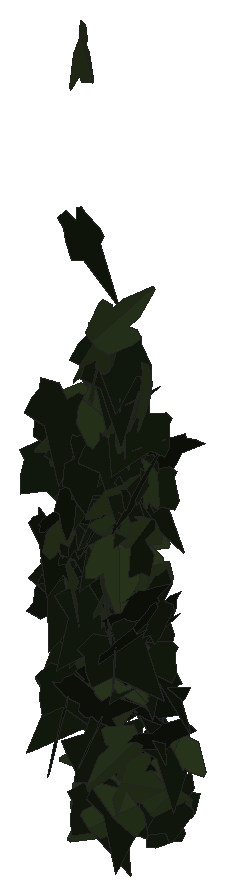
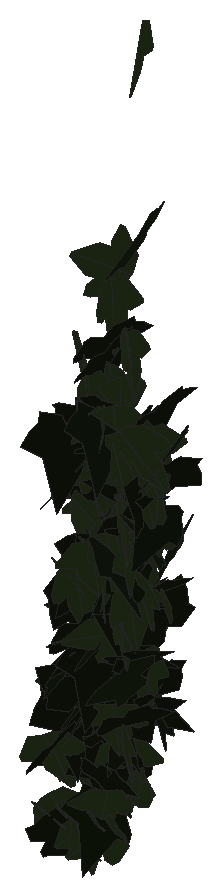
# SketchUp Ruby script. Lengths in inches.
U = 1.inch
M = Sketchup.active_model
def pt(a) = Geom::Point3d.new(a.map { |v| v * U })
def face(e, loops, mat)
  f = e.add_face(loops[0].map { |a| pt(a) })
  loops[1..].each { |l| e.add_face(l.map { |a| pt(a) }).erase! }
  f.material = f.back_material = mat if mat
  f
end
# faces: each face lists its corners as indices into pts; further lists are holes
def faces(e, pts, list, mat = nil) = list.each { |f| face(e, (f[0].is_a?(Array) ? f : [f]).map { |l| l.map { |i| pts[i] } }, mat) }
# xy, xz, yz: faces in a plane at the given z, y or x. An outline is a flat list of corners, or four numbers for a rectangle; further outlines are holes
def ring(l) = l.size == 4 ? [[l[0], l[1]], [l[2], l[1]], [l[2], l[3]], [l[0], l[3]]] : l.each_slice(2).to_a
def flat(e, list, mat, &to3) = list.each { |f| face(e, (f[0].is_a?(Array) ? f : [f]).map { |l| ring(l).map { |u, v| to3.(u, v) } }, mat) }
def xy(e, z, list, mat = nil) = flat(e, list, mat) { |x, y| [x, y, z] }
def xz(e, y, list, mat = nil) = flat(e, list, mat) { |x, z| [x, y, z] }
def yz(e, x, list, mat = nil) = flat(e, list, mat) { |y, z| [x, y, z] }
def lines(e, pts, list) = list.each { |a, b| e.add_line(pt(pts[a]), pt(pts[b])) }
# prism: a flat outline (further loops are holes) pulled along v
def prism(e, loops, v, mat = nil)
  f = face(e, loops, mat); d = Geom::Vector3d.new(v.map { |x| x * U })
  f.pushpull(f.normal.samedirection?(d) ? d.length : -d.length)
end
def box(e, o, s, mat = nil) = prism(e, [[o, [o[0] + s[0], o[1], o[2]], [o[0] + s[0], o[1] + s[1], o[2]], [o[0], o[1] + s[1], o[2]]]], [0, 0, s[2]], mat)
def at(x, y, z, deg = 0) = Geom::Transformation.translation(pt([x, y, z])) * Geom::Transformation.rotation(ORIGIN, Z_AXIS, deg.degrees)
def axes(o, x, y, z) = Geom::Transformation.new([*x, 0, *y, 0, *z, 0, *pt(o).to_a, 1])
def part(name) = M.definitions.add(name)
# library, detail: a bought-in or finely detailed component or shape, given as its bounding box
def library(name, o, s) = part(name).tap { |d| box(d.entities, o, s) }
def detail(e, o, s) = box(e.add_group.entities, o, s)
def put(e, d, t, mat = nil) = e.add_instance(d, t).tap { |i| i.material = mat if mat }
def group(e, t, mat = nil) = e.add_group.tap { |g| g.transformation = t; g.material = mat if mat }.entities
root = M.entities
M.materials.add("efeu1").color = [18, 25, 13]
M.materials.add("efeu2").color = [43, 57, 29]
c1 = part("ivyleaf_10")
p = [[0,0.5,-0.03],[-0.0625,2.02,-0.43],[-0.19,2.01,-0.46],[-0.54,1.05,-0.29],[-0.52,0.625,-0.18],[-0.83,0.76,-0.28],
  [-1.16,0.64,-0.33],[-1.15,0.33,-0.24],[-0.77,-0.39,0.02],[-0.3,-0.51,0.16],[0.04,-0.48,0.23],[-0.02,2.01,-0.4375],
  [-0.06,2.01,-0.43],[0.04,-0.49,0.23],[0.67,-0.49,0.14],[1.38,0.36,-0.2],[1.375,0.51,-0.24],[0.81,0.65,-0.19],
  [0.62,0.59,-0.15],[0.6,1.09,-0.28],[0.5,1.23,-0.31]]
faces(c1.entities,p,[[0,1,2,3,4,5,6,7,8,9,10],[11,12,0,13,14,15,16,17,18,19,20]],"efeu2")
c2 = part("ivyleaf_9")
p = [[1.54,2.16,1.25],[1.36,2.04,1.19],[-0.21,0.99,0.68],[-0.71,1.11,0.82],[-0.85,0.86,0.67],[-0.8,0.17,0.21],
  [-0.9,-0.01,0.1],[-0.67,-0.16,-0.02],[-0.08,-0.08,-0.05],[-0.03,-0.6,-0.4],[0.65,-0.88,-0.66],[0.83,-0.6,-0.49],
  [1.29,-0.42,-0.43],[1.8125,-0.07,-0.26],[1.21,0.44,0.15]]
faces(c2.entities,p,[[0,1,2,3,4,5,6,7,8,9,10,11,12,13,14]],"efeu1")
put(root,c1,axes([544.36,133.63,215.28],[0.76593,-0.47573,-0.00913],[0.0013,0.0194,-0.90149],[0.47582,0.76574,0.01717]))
put(root,c2,axes([544.35,134.4,210.57],[-0.44146,-0.74203,-0.00391],[0.04769,-0.02384,-0.86178],[0.7405,-0.44083,0.05318]))
put(root,c2,axes([543.96,132.84,219.55],[0.33357,-0.84112,0.18283],[0.07333,-0.16759,-0.90483],[0.85763,0.34148,0.00626]))
put(root,c1,axes([544.5625,133.91,214.71],[-0.18396,-0.86827,0.02169],[0.00495,-0.02321,-0.8875],[0.86853,-0.18377,0.00965]))
put(root,c2,axes([543.97,134.21,212.19],[0.76378,-0.42176,-0.05989],[0.10196,0.30037,-0.81499],[0.41361,0.70479,0.3115]))
put(root,c2,axes([544.15,132.43,215.58],[0.12089,-0.66184,0.61024],[0.07547,-0.6061,-0.6723],[0.89706,0.14019,-0.02568]))
put(root,c1,axes([544.85,133.55,220.17],[0.81777,0.15887,-0.54508],[-0.54725,-0.03404,-0.83094],[-0.15124,0.98219,0.05937]))
put(root,c2,axes([544.77,133.875,212.46],[-0.69047,-0.50333,0.18217],[-0.01066,-0.28433,-0.82602],[0.53518,-0.65505,0.21857]))
put(root,c2,axes([544.31,132.46,213.21],[-0.08317,-0.27642,0.86094],[0.76205,0.44397,0.21616],[-0.48674,0.74232,0.19131]))
put(root,c2,axes([544.72,132,217.1],[0.19383,0.78185,0.38972],[0.11374,0.37321,-0.8053],[-0.86616,0.22397,-0.01854]))
put(root,c1,axes([544.78,132.54,219.66],[-0.17417,-0.89754,0.09825],[-0.02854,-0.09454,-0.91423],[0.90245,-0.17621,-0.00995]))
put(root,c1,axes([544.98,132.62,211.78],[-0.85614,0.15785,0.30309],[-0.30004,0.04409,-0.87051],[-0.16356,-0.90713,0.01043]))
put(root,c2,axes([544.85,132.92,217.6],[0.05782,-0.11447,0.88511],[0.12882,0.87875,0.10523],[-0.88314,0.12069,0.0733]))
put(root,c2,axes([544.96,132.96,210.1],[-0.67636,-0.5024,0.20746],[-0.15286,-0.142,-0.84225],[0.52161,-0.69307,0.02218]))
put(root,c2,axes([544.39,132.33,218.87],[-0.09644,-0.71579,-0.59865],[0.14264,0.58346,-0.7206],[0.92217,-0.1651,0.04886]))
put(root,c1,axes([545.19,132.8,218.66],[-0.80348,-0.04527,0.45626],[-0.45087,-0.08926,-0.80284],[0.08331,-0.91966,0.05546]))
put(root,c2,axes([544.6875,132.9,214.22],[-0.29914,-0.82493,0.19051],[-0.01884,-0.19552,-0.87618],[0.84643,-0.29589,0.04783]))
put(root,c1,axes([544.74,132.17,216.39],[-0.06668,-0.76893,-0.42899],[0.26526,0.39269,-0.7451],[0.8396,-0.18513,0.20133]))
put(root,c2,axes([544.6875,132.37,210.19],[-0.42072,0.13063,-0.75248],[0.69411,-0.29297,-0.43895],[-0.31859,-0.8108,0.03738]))
put(root,c1,axes([544.93,133.96,209.78],[0.67624,-0.5645,-0.16398],[-0.10467,0.13032,-0.88029],[0.57844,0.68352,0.03241]))
put(root,c1,axes([544.78,134.39,210.59],[0.72269,0.46259,-0.0301],[-0.0271,-0.01349,-0.85806],[-0.46278,0.72319,0.00324]))
put(root,c1,axes([545.02,133.05,219.49],[-0.07678,-0.81983,0.38889],[-0.01917,-0.38872,-0.82327],[0.90718,-0.0776,0.01552]))
put(root,c2,axes([544.48,133.22,215.6875],[0.42107,-0.79258,-0.01396],[-0.01076,0.01009,-0.89748],[0.79263,0.42118,-0.00476]))
put(root,c1,axes([545,133.44,215.64],[-0.05752,-0.87897,-0.07927],[0.02266,0.07794,-0.88067],[0.88224,-0.05931,0.01745]))
put(root,c2,axes([544.74,132.31,211.1875],[0.10884,-0.57616,-0.64225],[-0.1346,0.62808,-0.58625],[0.85225,0.17278,-0.01057]))
put(root,c2,axes([544.75,132.31,220.81],[-0.04428,-0.92209,0.0919],[-0.01273,-0.09139,-0.92311],[0.92657,-0.04532,-0.00829]))
put(root,c1,axes([545.08,133.77,213.84],[0.26784,-0.85015,-0.09039],[-0.00354,0.09362,-0.89101],[0.85494,0.26673,0.02463]))
put(root,c1,axes([545.17,133.41,217.6],[0.24785,-0.82408,-0.29428],[-0.06142,0.28872,-0.86024],[0.87289,0.25431,0.02303]))
put(root,c2,axes([545.22,134.38,206.92],[0.27446,0.78455,0.18613],[-0.04767,0.21206,-0.82356],[-0.80492,0.25496,0.11224]))
put(root,c2,axes([545.52,133.95,216.19],[-0.56786,0.67413,-0.07436],[0.03608,-0.06682,-0.88129],[-0.67726,-0.56879,0.01539]))
put(root,c2,axes([544.86,132.83,212.32],[0.00984,-0.18546,0.87666],[0.64093,0.61414,0.12273],[-0.6262,0.62567,0.13939]))
put(root,c1,axes([544.58,132.39,214.32],[0.57667,-0.23355,0.67278],[0.65854,-0.15469,-0.61816],[0.27112,0.8725,0.07049]))
put(root,c2,axes([545.32,132.11,215.97],[-0.64082,0.64069,-0.17112],[-0.15267,0.08903,0.90508],[0.64533,0.65727,0.0442]))
put(root,c2,axes([544.84,133.26,215.51],[0.87645,-0.01594,-0.19155],[-0.18917,0.08691,-0.8728],[0.03406,0.89292,0.08154]))
put(root,c2,axes([545.02,133.65,217.5],[-0.25745,-0.84777,0.09368],[-0.01198,-0.09425,-0.88586],[0.85285,-0.25724,0.01584]))
put(root,c2,axes([545.25,134.58,208.4],[-0.7727,-0.20546,-0.31245],[0.30923,0.05222,-0.7991],[0.21027,-0.83184,0.02701]))
put(root,c1,axes([544.95,134.63,207.49],[0.53789,0.64418,0.14873],[0.10208,0.10851,-0.83917],[-0.65319,0.54742,-0.00867]))
put(root,c1,axes([544.96,133.61,215.96],[-0.64233,0.37563,-0.49597],[0.39211,-0.30905,-0.74189],[-0.48304,-0.75037,0.05728]))
put(root,c1,axes([545.02,132.83,217.82],[0.8416,0.13114,0.2751],[0.22307,0.28542,-0.8185],[-0.20765,0.83816,0.23568]))
put(root,c2,axes([545.33,133.57,213.62],[-0.48779,-0.73922,0.07842],[-0.02927,-0.07463,-0.8855],[0.74279,-0.48838,0.01661]))
put(root,c2,axes([545.74,132.59,209.23],[-0.31755,0.22971,-0.89619],[-0.69468,0.56659,0.39137],[0.61103,0.76353,-0.0208]))
put(root,c1,axes([544.91,134.52,206.15],[0.4604,0.15133,0.70044],[0.55774,0.44707,-0.46319],[-0.44994,0.70902,0.14256]))
put(root,c1,axes([545.67,132.85,208.19],[-0.68468,-0.53058,0.13792],[-0.10141,-0.09429,-0.86611],[0.53875,-0.69204,0.01226]))
put(root,c1,axes([545.51,133.18,219.44],[0.18367,-0.89419,-0.13502],[0.05585,0.14873,-0.90901],[0.9026,0.17275,0.08372]))
put(root,c1,axes([545.12,133.69,213.18],[0.01221,-0.03147,0.96719],[0.33212,0.90866,0.02537],[-0.90893,0.33159,0.02227]))
put(root,c1,axes([545.63,133.72,216.64],[-0.16809,-0.88289,0.05335],[0.01245,-0.05667,-0.89846],[0.88441,-0.167,0.02279]))
put(root,c2,axes([545.45,132.96,219.14],[-0.38516,-0.83459,-0.0298],[0.01269,0.02697,-0.91918],[0.83502,-0.38537,0.00022]))
put(root,c2,axes([545.62,131.37,218.44],[0.3081,-0.25107,-0.81837],[-0.6012,0.55569,-0.39683],[0.60937,0.67519,0.02227]))
put(root,c2,axes([545.125,132.46,227.24],[0.61678,-0.73433,-0.17989],[-0.108,0.1442,-0.95893],[0.74829,0.62608,0.00987]))
put(root,c1,axes([545.7,132.54,223.06],[0.2438,-0.87203,-0.24082],[-0.08085,0.22741,-0.90533],[0.90105,0.25635,-0.01607]))
put(root,c1,axes([545.63,131.91,234.07],[0.36414,-0.78088,-0.4151],[0.10064,0.48258,-0.81955],[0.87861,0.26836,0.26591]))
put(root,c2,axes([545.84,133.86,212.04],[0.23782,0.83183,0.02298],[-0.00237,0.02458,-0.86511],[-0.83214,0.23766,0.00903]))
put(root,c1,axes([545.84,134.55,206.27],[-0.0782,-0.85343,0.02497],[0.02324,-0.0272,-0.85662],[0.85348,-0.07745,0.02561]))
put(root,c1,axes([545.81,133.34,214.16],[0.23315,-0.83809,-0.10634],[0.02832,0.118,-0.86795],[0.84433,0.22747,0.05847]))
put(root,c2,axes([546.08,133.49,220.29],[0.00529,0.86938,0.22364],[-0.0784,0.22324,-0.86596],[-0.89425,-0.01443,0.07724]))
put(root,c2,axes([545.74,132.6875,213.41],[-0.33371,-0.69729,0.46265],[-0.09182,-0.46456,-0.76641],[0.83177,-0.33105,0.10102]))
put(root,c1,axes([545.87,133.11,220.43],[-0.72833,-0.53396,0.11151],[0.07158,-0.27797,-0.86349],[0.54076,-0.68237,0.26449]))
put(root,c2,axes([545.9,133.74,211.04],[-0.33829,0.38007,-0.70218],[0.40763,-0.57352,-0.50682],[-0.68654,-0.5278,0.04508]))
put(root,c1,axes([545.52,132.9,207.07],[0.66572,0.44384,0.35574],[0.28348,0.21589,-0.79985],[-0.49314,0.72327,0.02045]))
put(root,c2,axes([546.15,133.11,208.21],[0.36892,0.61662,-0.44663],[-0.32938,-0.31821,-0.71138],[-0.68645,0.48408,0.1013]))
put(root,c1,axes([545.53,132.89,207.15],[0.44954,0.52465,0.53791],[0.33224,0.42344,-0.69066],[-0.67396,0.55869,0.01832]))
put(root,c2,axes([546.01,133.65,216.38],[-0.68444,-0.58294,0.0227],[0.09911,-0.15067,-0.88107],[0.57491,-0.66804,0.1789]))
put(root,c1,axes([545.4,134.88,206.39],[0.49585,0.16725,0.65925],[0.61367,0.24174,-0.5229],[-0.29324,0.78869,0.02047]))
put(root,c1,axes([545.33,132.62,216.61],[-0.24732,-0.03994,0.91667],[0.90806,0.12549,0.25047],[-0.13157,0.94112,0.0055]))
put(root,c2,axes([546.24,132.4,208.35],[-0.526,-0.50541,0.58798],[0.42046,0.41104,0.72945],[-0.65144,0.67339,-0.00395]))
put(root,c1,axes([546.06,133.97,215.94],[0.58512,0.65554,-0.11344],[-0.14178,-0.02474,-0.87422],[-0.65,0.59551,0.08856]))
put(root,c1,axes([545.96,132.18,221.1],[0.01216,0.69272,0.62534],[0.03582,0.62458,-0.69259],[-0.93254,0.03303,-0.01845]))
put(root,c1,axes([546.17,132.04,222.82],[0.50566,-0.74084,-0.2527],[-0.04956,0.26994,-0.89055],[0.78118,0.49667,0.10708]))
put(root,c2,axes([545.81,133.875,210.78],[0.50991,-0.59501,-0.36846],[-0.20506,0.30886,-0.78254],[0.66914,0.54807,0.04097]))
put(root,c2,axes([545.72,133.33,217.41],[0.47746,-0.77371,-0.06069],[-0.03173,0.05174,-0.90917],[0.77544,0.47852,0.00016]))
put(root,c2,axes([546.03,131.29,219.61],[0.49181,-0.18705,-0.77102],[-0.45525,0.6764,-0.45448],[0.64977,0.61549,0.26515]))
put(root,c2,axes([545.47,132.2,210.34],[0.2158,-0.27569,0.81243],[0.77852,-0.28908,-0.30489],[0.36049,0.78933,0.17209]))
put(root,c2,axes([545.71,133.96,212.89],[0.54656,-0.69755,0.00833],[0.07901,0.05138,-0.88119],[0.69311,0.5442,0.09387]))
put(root,c2,axes([545.91,132.48,207.05],[0.23239,-0.8098,-0.40261],[-0.05992,0.40098,-0.84113],[0.90237,0.23517,0.04782]))
put(root,c1,axes([546.16,133.6,219.99],[-0.59001,0.63296,-0.23476],[0.16978,-0.16263,-0.86521],[-0.6534,-0.61382,-0.01284]))
put(root,c1,axes([546.38,132.43,221.52],[0.78496,-0.42416,-0.25464],[-0.14588,0.2579,-0.87927],[0.47273,0.78389,0.15149]))
put(root,c2,axes([545.69,132.29,211.11],[0.91705,0.06919,0.33829],[0.33798,0.01671,-0.91962],[-0.0707,0.97732,-0.00823]))
put(root,c2,axes([546.65,133.53,217.85],[-0.82235,-0.36882,0.08779],[-0.03618,-0.13238,-0.89508],[0.37739,-0.81636,0.10548]))
put(root,c1,axes([546.46,132.91,218.52],[-0.25498,-0.87423,0.02858],[0.04245,-0.04211,-0.90914],[0.87367,-0.2531,0.05252]))
put(root,c1,axes([546.64,132.71,211.03],[-0.74081,-0.38851,0.17924],[-0.14312,-0.11272,-0.83587],[0.40322,-0.7538,0.03261]))
put(root,c2,axes([546.97,135.08,205.47],[-0.23465,-0.01298,0.79596],[-0.74222,-0.29644,-0.22364],[0.2878,-0.77507,0.0722]))
put(root,c2,axes([547.02,132.91,219],[-0.79087,-0.15544,0.42751],[-0.39164,-0.20346,-0.7985],[0.23138,-0.87569,0.10964]))
put(root,c2,axes([546.11,133.23,216.77],[0.28305,-0.83105,0.13109],[0.05584,-0.11945,-0.87782],[0.83947,0.28815,0.01419]))
put(root,c2,axes([546.37,132.87,223.18],[-0.21484,-0.9064,-0.06104],[-0.00127,0.06302,-0.93138],[0.90846,-0.21427,-0.01574]))
put(root,c1,axes([547.1,132.24,207],[-0.41534,-0.28419,0.85261],[-0.58353,-0.62908,-0.49394],[0.68352,-0.70973,0.09641]))
put(root,c1,axes([546.04,132.58,214.34],[0.23839,-0.32064,0.81146],[0.7134,-0.41267,-0.37265],[0.50233,0.73824,0.14413]))
put(root,c2,axes([546.47,134.05,213.17],[-0.33825,-0.8139,0.00539],[0.00067,-0.00611,-0.88138],[0.81392,-0.33823,0.00296]))
put(root,c1,axes([547.03,134.63,206.52],[-0.56494,-0.36197,0.49649],[-0.4185,-0.26714,-0.67095],[0.44987,-0.70306,-0.00068]))
put(root,c1,axes([546.6,133.09,220.38],[-0.12147,0.88578,-0.09809],[0.00937,-0.09773,-0.89406],[-0.89114,-0.12177,0.00397]))
put(root,c2,axes([546.41,132.84,222.61],[0.06897,-0.93395,0.015],[-0.02185,-0.01665,-0.93621],[0.93381,0.06859,-0.02301]))
put(root,c1,axes([546.83,133.82,214.72],[-0.36111,-0.80854,0.10452],[0.01601,-0.12133,-0.88322],[0.81511,-0.35582,0.06366]))
put(root,c1,axes([546.91,131.94,212.92],[0.45922,-0.45406,-0.66565],[-0.22043,0.66614,-0.60647],[0.77503,0.4585,0.22193]))
put(root,c1,axes([546.85,131.88,224.15],[-0.02183,-0.91782,-0.19191],[-0.00652,0.19211,-0.91801],[0.93764,-0.02003,-0.01086]))
put(root,c2,axes([546.33,134.19,210.27],[0.36969,-0.78355,0.06825],[0.03031,-0.06116,-0.86639],[0.78593,0.37093,0.00131]))
put(root,c2,axes([546.45,134.06,212.16],[0.10354,-0.87319,-0.05486],[0.00059,0.05531,-0.87928],[0.87492,0.1033,0.00709]))
put(root,c1,axes([546.9,132.97,221.08],[0.01605,-0.91915,-0.05234],[-0.02662,0.05186,-0.91893],[0.92025,0.01753,-0.02567]))
put(root,c2,axes([546.62,132.85,219.69],[-0.18883,-0.89614,-0.10866],[0.04089,0.10241,-0.91563],[0.90178,-0.19229,0.01876]))
put(root,c2,axes([547.06,133.44,220.64],[-0.753,-0.51193,0.01515],[-0.00835,-0.01465,-0.91051],[0.51209,-0.75301,0.00742]))
put(root,c2,axes([547.4,134.8,206.25],[-0.79437,0.24896,0.09282],[-0.1168,-0.06438,-0.82694],[-0.23865,-0.79718,0.09577]))
put(root,c2,axes([546.6,132.8,206.94],[0.03891,-0.8499,0.36099],[0.06337,-0.35801,-0.84969],[0.92121,0.06053,0.04321]))
put(root,c1,axes([547.04,132.23,218.4],[-0.25902,-0.88105,-0.13872],[0.03394,0.13461,-0.91832],[0.89126,-0.26118,-0.00534]))
put(root,c2,axes([547.04,133.86,212.3],[-0.50278,-0.65718,0.26594],[-0.03391,-0.30336,-0.81377],[0.70814,-0.48112,0.14984]))
put(root,c1,axes([547.09,132.47,209.21],[-0.05305,-0.36828,0.84343],[0.06482,-0.84423,-0.36455],[0.91804,0.03833,0.07448]))
put(root,c2,axes([546.93,133.45,210.1],[0.72587,0.26863,0.52476],[-0.49818,-0.16555,0.77385],[0.31521,-0.88026,0.0146]))
put(root,c2,axes([547.875,132.23,217.05],[-0.4684,-0.04706,-0.80742],[-0.74861,-0.32794,0.4534],[-0.30613,0.87395,0.12666]))
put(root,c1,axes([546.79,132.01,212.3],[0.29861,0.64093,0.53578],[0.25151,0.47361,-0.70673],[-0.79662,0.38978,-0.02229]))
put(root,c1,axes([547.01,133.4,217.04],[0.23732,-0.66291,0.5677],[0.20957,-0.52782,-0.70395],[0.84724,0.31625,0.01511]))
put(root,c2,axes([547.22,133.45,218.67],[-0.53956,-0.73118,0.03863],[-0.0173,-0.03523,-0.90868],[0.73199,-0.53979,0.00699]))
put(root,c2,axes([546.92,131.9375,212.55],[0.38952,0.07196,0.79449],[0.48705,0.67878,-0.30027],[-0.63181,0.56763,0.25835]))
put(root,c2,axes([547.41,133.5,219.55],[0.32494,0.83188,-0.10686],[-0.10054,-0.07514,-0.89066],[-0.83266,0.3337,0.06584]))
put(root,c1,axes([547.16,132.4375,207.97],[-0.08346,-0.44258,-0.76989],[0.26436,0.72584,-0.44592],[0.84777,-0.26991,0.06326]))
put(root,c1,axes([547.54,132.07,217.48],[-0.71668,-0.53487,0.18646],[-0.15418,-0.10514,-0.89423],[0.54505,-0.73304,-0.00779]))
put(root,c2,axes([546.98,131.83,213.3],[0.10158,-0.50291,-0.73544],[0.04677,0.74219,-0.50107],[0.88972,0.0184,0.11031]))
put(root,c2,axes([547.58,133.15,209.53],[0.13095,0.85091,-0.23638],[-0.07352,-0.22764,-0.86015],[-0.88007,0.14563,0.03668]))
put(root,c2,axes([547.26,131.73,217.75],[-0.38172,0.85567,0.03737],[0.01027,-0.03634,0.93694],[0.85642,0.38182,0.00542]))
put(root,c2,axes([547.32,132.05,214.41],[0.37622,0.72103,0.35586],[0.15349,0.32126,-0.8132],[-0.78928,0.40617,0.01148]))
put(root,c1,axes([547.21,131.25,224.65],[-0.0733,-0.57656,0.80241],[0.07704,0.79883,0.58102],[-0.98506,0.10538,-0.01427]))
put(root,c2,axes([547.58,133.34,213.88],[-0.327,0.59599,-0.5634],[0.25687,-0.50159,-0.67969],[-0.77887,-0.41565,0.01238]))
put(root,c2,axes([547.8,133.3,214.29],[-0.83866,0.2784,-0.06454],[0.05937,-0.026,-0.88364],[-0.27955,-0.84074,0.00596]))
put(root,c1,axes([547.34,132.95,218.78],[0.84413,-0.30051,-0.03469],[-0.03191,0.01379,-0.89603],[0.30082,0.84473,0.00229]))
put(root,c1,axes([547.48,134.37,208.53],[0.73607,0.34389,-0.30202],[-0.29364,-0.08389,-0.81118],[-0.35107,0.79119,0.04526]))
put(root,c1,axes([547.24,131.84,216.6],[0.56927,0.81098,-0.01658],[-0.01133,-0.0123,-0.99084],[-0.81107,0.56938,0.00221]))
put(root,c2,axes([547.17,134.6,208.68],[0.07984,-0.84584,0.09159],[-0.00649,-0.0926,-0.84946],[0.85076,0.07868,-0.01507]))
put(root,c2,axes([546.97,134.13,211.53],[0.48891,-0.7024,0.1556],[0.09899,-0.12067,-0.85572],[0.71259,0.49868,0.01211]))
put(root,c2,axes([547.09,133,218.47],[0.53064,-0.66287,-0.33758],[-0.09617,0.35005,-0.83854],[0.73764,0.52249,0.13352]))
put(root,c1,axes([547.77,132.55,222.23],[0.41088,-0.60071,-0.54336],[-0.30545,0.44938,-0.72778],[0.75019,0.51197,0.00127]))
